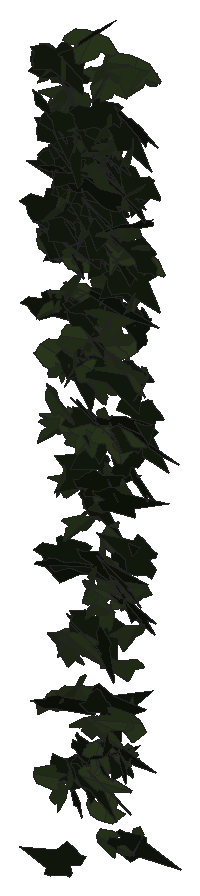
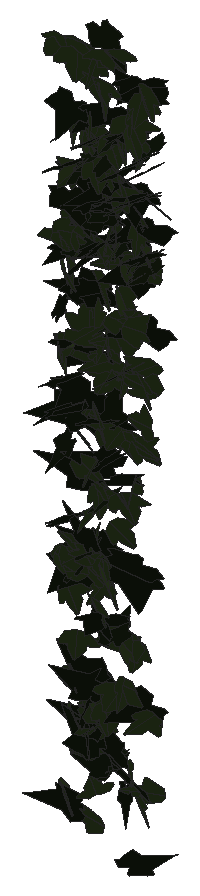
# SketchUp Ruby script. Lengths in millimetres.
U = 1.mm
M = Sketchup.active_model
def pt(a) = Geom::Point3d.new(a.map { |v| v * U })
def face(e, loops, mat)
  f = e.add_face(loops[0].map { |a| pt(a) })
  loops[1..].each { |l| e.add_face(l.map { |a| pt(a) }).erase! }
  f.material = f.back_material = mat if mat
  f
end
# faces: each face lists its corners as indices into pts; further lists are holes
def faces(e, pts, list, mat = nil) = list.each { |f| face(e, (f[0].is_a?(Array) ? f : [f]).map { |l| l.map { |i| pts[i] } }, mat) }
# xy, xz, yz: faces in a plane at the given z, y or x. An outline is a flat list of corners, or four numbers for a rectangle; further outlines are holes
def ring(l) = l.size == 4 ? [[l[0], l[1]], [l[2], l[1]], [l[2], l[3]], [l[0], l[3]]] : l.each_slice(2).to_a
def flat(e, list, mat, &to3) = list.each { |f| face(e, (f[0].is_a?(Array) ? f : [f]).map { |l| ring(l).map { |u, v| to3.(u, v) } }, mat) }
def xy(e, z, list, mat = nil) = flat(e, list, mat) { |x, y| [x, y, z] }
def xz(e, y, list, mat = nil) = flat(e, list, mat) { |x, z| [x, y, z] }
def yz(e, x, list, mat = nil) = flat(e, list, mat) { |y, z| [x, y, z] }
def lines(e, pts, list) = list.each { |a, b| e.add_line(pt(pts[a]), pt(pts[b])) }
# prism: a flat outline (further loops are holes) pulled along v
def prism(e, loops, v, mat = nil)
  f = face(e, loops, mat); d = Geom::Vector3d.new(v.map { |x| x * U })
  f.pushpull(f.normal.samedirection?(d) ? d.length : -d.length)
end
def box(e, o, s, mat = nil) = prism(e, [[o, [o[0] + s[0], o[1], o[2]], [o[0] + s[0], o[1] + s[1], o[2]], [o[0], o[1] + s[1], o[2]]]], [0, 0, s[2]], mat)
def at(x, y, z, deg = 0) = Geom::Transformation.translation(pt([x, y, z])) * Geom::Transformation.rotation(ORIGIN, Z_AXIS, deg.degrees)
def axes(o, x, y, z) = Geom::Transformation.new([*x, 0, *y, 0, *z, 0, *pt(o).to_a, 1])
def part(name) = M.definitions.add(name)
# library, detail: a bought-in or finely detailed component or shape, given as its bounding box
def library(name, o, s) = part(name).tap { |d| box(d.entities, o, s) }
def detail(e, o, s) = box(e.add_group.entities, o, s)
def put(e, d, t, mat = nil) = e.add_instance(d, t).tap { |i| i.material = mat if mat }
def group(e, t, mat = nil) = e.add_group.tap { |g| g.transformation = t; g.material = mat if mat }.entities
root = M.entities
M.materials.add("efeu1").color = [18, 25, 13]
M.materials.add("efeu2").color = [43, 57, 29]
c1 = part("ivyleaf_9")
p = [[39.1,54.8,31.7],[34.5,51.8,30.2],[-5.3,25.2,17.3],[-17.9,28.3,20.9],[-21.6,21.7,17],[-20.2,4.3,5.3],
  [-22.9,-0.3,2.5],[-17.1,-4,-0.6],[-2,-2.1,-1.2],[-0.7,-15.4,-10.1],[16.6,-22.3,-16.7],[21.1,-15.1,-12.5],
  [32.7,-10.7,-11],[46.1,-1.8,-6.6],[30.8,11.2,3.8]]
faces(c1.entities,p,[[0,1,2,3,4,5,6,7,8,9,10,11,12,13,14]],"efeu1")
c2 = part("ivyleaf_10")
p = [[0,12.8,-0.8],[-1.5,51.3,-10.9],[-4.9,51,-11.6],[-13.6,26.5,-7.3],[-13.2,15.9,-4.6],[-21.1,19.3,-7.2],
  [-29.5,16.3,-8.3],[-29.2,8.3,-6.2],[-19.7,-9.8,0.5],[-7.6,-13,4],[1,-12.2,5.8],[-0.4,51.1,-11.1],
  [-1.5,51.1,-10.9],[1,-12.4,5.9],[16.9,-12.4,3.5],[35.1,9.1,-5.1],[35,12.9,-6.1],[20.5,16.4,-4.9],
  [15.8,15,-3.8],[15.3,27.6,-7.1],[12.8,31.3,-7.8]]
faces(c2.entities,p,[[0,1,2,3,4,5,6,7,8,9,10],[11,12,0,13,14,15,16,17,18,19,20]],"efeu2")
put(root,c1,axes([2017.3,949.6,846.8],[0.22313,0.05004,0.79873],[1.37801,0.33725,-0.12741],[-0.64884,0.73347,0.00409]))
put(root,c2,axes([2051.2,960.3,1148.2],[-1.33642,-0.23546,0.06145],[-0.10791,-0.0242,-0.74061],[0.45038,-0.70447,0.00491]))
put(root,c2,axes([2099.1,965.4,1580.9],[-1.10747,-0.55056,0.2142],[-0.17202,-0.21415,-0.79598],[1.11111,-0.58192,0.09026]))
put(root,c2,axes([2088.2,957.8,1448.8],[0.19663,-0.77036,-0.31589],[0.05218,0.32128,-0.77456],[1.58377,0.08505,0.06474]))
put(root,c2,axes([1923,963.4,1232.1],[-0.03515,-0.04676,0.81979],[1.56112,0.03653,0.02056],[-0.07163,0.81918,0.04588]))
put(root,c1,axes([1995,969.1,336.1],[0.64527,-0.78076,0.06942],[0.0749,-0.05858,-0.85111],[1.48993,0.34108,0.01272]))
put(root,c2,axes([1955,966.6,1335.6],[0.91903,-0.61856,0.09808],[0.10345,-0.08199,-0.78469],[1.18745,0.48588,-0.00755]))
put(root,c2,axes([2072.5,963.3,1299.6],[-0.8108,-0.67903,0.04435],[-0.04819,-0.03647,-0.8016],[1.29418,-0.42676,-0.00206]))
put(root,c2,axes([2086.8,962.5,459.6],[0.64898,-0.00928,-0.69136],[-1.3048,0.09545,-0.33942],[0.17068,0.76495,0.03397]))
put(root,c1,axes([2016.9,971.5,582.5],[-0.39013,0.04915,-0.84771],[1.57044,-0.19423,-0.2108],[-0.38131,-0.85024,-0.00085]))
put(root,c2,axes([2013.5,964.2,432],[-0.80071,0.13176,-0.54735],[0.98165,-0.18367,-0.44067],[-0.42945,-0.66548,0.01325]))
put(root,c1,axes([2055.7,980,1208.8],[0.36229,-0.31801,-0.71542],[0.61667,-0.63825,0.36992],[-1.35645,-0.3751,-0.02291]))
put(root,c2,axes([2037.4,962.1,1436.9],[-0.52323,-0.77628,-0.1375],[0.09712,0.12779,-0.82351],[1.49727,-0.27956,0.00536]))
put(root,c1,axes([2008.8,973.2,945.6],[1.07179,-0.67128,0.12791],[-0.10135,0.12214,0.87542],[-1.29661,-0.56443,0.03731]))
put(root,c2,axes([1942.4,973.1,919.2],[-0.2544,-0.58614,0.47424],[-0.23255,-0.45842,-0.60103],[1.41597,-0.1806,-0.01351]))
put(root,c1,axes([1949.1,957.5,1529.6],[-0.86966,-0.09896,0.70036],[1.33591,0.03932,0.46352],[-0.16592,0.83532,0.06115]))
put(root,c1,axes([2004.6,963.6,1339.3],[0.22572,-0.16988,0.8106],[1.48383,-0.25337,-0.16717],[0.53179,0.77907,0.12239]))
put(root,c1,axes([1980.2,966.9,1133.4],[0.57441,-0.71253,-0.15559],[-0.05756,0.15602,-0.77314],[1.38685,0.30159,0.03235]))
put(root,c2,axes([1938.2,953.1,1054.1],[0.51783,0.45753,0.6261],[0.58708,0.5449,-0.53225],[-1.35405,0.41123,0.00867]))
put(root,c1,axes([1956.2,973.8,164.7],[-0.09001,-0.01374,0.76617],[-1.35631,-0.28136,-0.04904],[0.53606,-0.7142,0.00458]))
put(root,c2,axes([2007.8,958.4,340.2],[-0.27323,-0.14885,-0.75209],[1.39735,0.19361,-0.17847],[0.42011,-0.74078,0.10448]))
put(root,c1,axes([1983.4,974.7,1025.8],[-0.02468,-0.76983,0.10528],[-0.00828,-0.10522,-0.76993],[1.47875,-0.01344,-0.00255]))
put(root,c1,axes([1943.6,963.3,1565.4],[-0.2483,-0.62877,-0.56176],[0.14015,0.55778,-0.64141],[1.59858,-0.14656,-0.03102]))
put(root,c1,axes([2040.6,971.7,474.3],[-0.10227,-0.21449,0.73979],[1.00549,-0.54991,-0.12106],[1.06677,0.49777,0.18503]))
put(root,c1,axes([2002.5,975.7,1317.4],[0.41487,-0.64149,0.45015],[0.41534,-0.39907,-0.67437],[1.43249,0.30149,0.06516]))
put(root,c2,axes([1959.7,959.8,550.7],[-1.33318,0.37854,0.14958],[-0.25108,0.07051,-0.79623],[-0.73283,-0.71281,0.00068]))
put(root,c2,axes([1924.4,973.5,961.1],[0.23048,-0.23441,0.79724],[1.40468,-0.33987,-0.21204],[0.72674,0.73127,0.15701]))
put(root,c1,axes([1974,965.2,1275.6],[-0.38098,-0.57923,-0.54341],[0.42026,0.49772,-0.61187],[1.45199,-0.29604,0.03452]))
put(root,c1,axes([1915.1,977.1,1456.4],[0.2872,-0.68165,0.39536],[0.20986,-0.38032,-0.6978],[1.48498,0.18558,0.02215]))
put(root,c1,axes([1928.9,957.3,1309.3],[-0.00385,-0.34703,-0.79748],[0.39652,0.77407,-0.33738],[1.60704,-0.19182,0.08133]))
put(root,c2,axes([2004.8,974,926.9],[-0.48843,-0.595,0.42459],[-0.03561,-0.4445,-0.63422],[1.39071,-0.22035,0.13288]))
put(root,c2,axes([1978.2,952,1093.1],[-0.2951,-0.17635,-0.85934],[1.20506,0.5815,-0.23358],[1.15556,-0.65144,0.02413]))
put(root,c1,axes([2038.5,972.1,708],[0.68577,-0.65111,0.19844],[0.18153,-0.17402,-0.74416],[1.28269,0.37273,-0.00078]))
put(root,c1,axes([2059.5,977.7,1364.5],[0.17038,-0.6586,0.46324],[0.40942,-0.42959,-0.65233],[1.47676,0.19509,0.12741]))
put(root,c2,axes([1999.8,962.3,922.1],[0.98723,-0.29665,-0.41728],[-0.63076,0.25821,-0.59555],[0.7427,0.61362,0.04888]))
put(root,c1,axes([1974.7,958.9,1371.3],[-0.88416,0.53391,0.36751],[-0.53638,0.24078,-0.70607],[-1.11087,-0.54121,0.04842]))
put(root,c2,axes([1984.1,977.6,1327.7],[0.17658,-0.30387,0.75573],[1.04993,-0.53617,-0.28332],[1.14055,0.54062,0.1438]))
put(root,c2,axes([2052.2,965.3,943.1],[1.37774,0.28758,0.14692],[0.26326,0.04974,-0.77892],[-0.55538,0.73699,-0.00476]))
put(root,c1,axes([1939,952.2,451],[1.26595,0.38495,0.3228],[0.50845,0.18255,-0.76821],[-0.80974,0.71647,0.02229]))
put(root,c2,axes([2027.8,974,943],[0.36732,-0.19282,0.66763],[1.10294,-0.33772,-0.26507],[0.72987,0.60739,0.06456]))
put(root,c1,axes([2054.6,981.6,1238.4],[-0.1307,-0.54907,0.63036],[0.24748,-0.63181,-0.53616],[1.57164,0.05383,0.13685]))
put(root,c2,axes([1960.7,957.1,841.4],[0.15558,-0.60823,-0.51662],[0.22322,0.52284,-0.597],[1.50231,-0.0147,0.14221]))
put(root,c1,axes([2066.6,982,654.5],[-0.02983,-0.43981,0.68525],[0.02123,-0.68543,-0.43967],[1.54952,0.00093,0.01922]))
put(root,c1,axes([2023.6,963.3,1630.6],[-0.396,0.75605,-0.28918],[0.176,-0.27443,-0.78401],[-1.53049,-0.22718,-0.01533]))
put(root,c2,axes([2057.4,979.8,1260.9],[-0.16097,-0.55649,0.62678],[0.35005,-0.62693,-0.53181],[1.55633,0.08345,0.18444]))
put(root,c2,axes([2033.6,963,1378.6],[-1.4652,0.10412,0.33772],[-0.64465,0.01357,-0.77632],[-0.1919,-0.84057,0.0293]))
put(root,c1,axes([2053.6,975.7,1166.6],[-0.0147,-0.02878,-0.80378],[-0.64011,-0.73005,0.02937],[-1.39048,0.33638,-0.00502]))
put(root,c2,axes([2046.2,971.1,1434.8],[-0.00868,-0.80127,0.13001],[-0.03442,-0.12988,-0.8011],[1.54454,-0.0074,-0.01712]))
put(root,c2,axes([2083.9,969.9,615.8],[-0.41394,-0.75893,0.10008],[-0.0215,-0.10085,-0.7893],[1.45674,-0.21714,0.01679]))
put(root,c1,axes([2009.8,967.5,1446.6],[0.63071,-0.69883,-0.2613],[0.06158,0.29911,-0.75891],[1.41861,0.29771,0.14911]))
put(root,c2,axes([2044.7,972.4,1097.9],[-0.94798,-0.6166,-0.17507],[-0.20852,-0.13655,0.79266],[-1.20195,0.51001,0.00057]))
put(root,c2,axes([1977.5,974.3,1445.4],[0.46495,-0.70608,0.29635],[0.34947,-0.24797,-0.74219],[1.41486,0.29328,0.08593]))
put(root,c1,axes([1933.9,965.7,1240.9],[0.65194,-0.65099,-0.38619],[-0.27509,0.35984,-0.73478],[1.41407,0.37013,0.03511]))
put(root,c2,axes([1950.2,965.2,1035],[0.89916,-0.6454,-0.29145],[-0.28808,0.25022,-0.79948],[1.31661,0.49552,0.02411]))
put(root,c2,axes([1947.7,982,1130.8],[-0.13574,-0.4363,0.75754],[-0.22223,-0.74849,-0.44209],[1.64887,-0.1368,0.00278]))
put(root,c1,axes([2011.4,971.9,700.2],[0.48049,-0.22291,0.73659],[1.12002,-0.44362,-0.33595],[0.94382,0.63992,0.02368]))
put(root,c2,axes([1966.7,967.8,563.1],[-0.98505,0.14037,-0.65553],[1.19464,-0.18934,-0.53614],[-0.44803,-0.81348,0.01168]))
put(root,c1,axes([2025.3,974.1,1315],[-1.25694,-0.28531,-0.38832],[0.70404,0.12198,-0.71878],[0.58769,-0.75637,0.03056]))
put(root,c1,axes([2025.5,965.6,1163],[1.06675,-0.13073,0.50882],[0.92625,-0.15095,-0.5749],[0.37649,0.74181,-0.02732]))
put(root,c1,axes([1954.1,980.3,1238.6],[0.22312,-0.67059,0.38038],[0.08005,-0.37861,-0.68045],[1.46511,0.12281,-0.02075]))
put(root,c2,axes([1930.5,970.9,1266.9],[0.57811,-0.70834,0.0458],[0.04705,-0.03923,-0.77069],[1.35011,0.30468,0.00725]))
put(root,c1,axes([1968,960.2,1366.3],[0.96449,0.45524,-0.40751],[-0.73472,-0.17179,-0.672],[-0.90131,0.62719,0.11172]))
put(root,c1,axes([1983.6,975.7,1338.3],[-0.51996,-0.74959,-0.16478],[0.08137,0.15977,-0.79769],[1.45841,-0.27616,-0.01424]))
put(root,c2,axes([2010.3,965.5,1020.2],[-1.34199,0.14114,-0.10133],[0.1947,-0.00507,-0.71895],[-0.26728,-0.71235,-0.01496]))
put(root,c2,axes([2008.2,962.4,1043.4],[-0.62937,-0.33628,-0.58463],[1.0408,0.24739,-0.45163],[0.75127,-0.62446,0.13591]))
put(root,c1,axes([2074.6,965.2,1227.1],[0.05079,-0.53096,-0.58579],[0.14023,0.58524,-0.5271],[1.49813,-0.03678,0.0692]))
put(root,c1,axes([1966.2,965,1462.8],[0.24546,-0.58757,-0.57627],[0.02116,0.5845,-0.59347],[1.56619,0.08419,0.09833]))
put(root,c2,axes([2068.5,972,1046.7],[-1.36516,-0.11572,-0.25862],[-0.48066,-0.05795,0.7264],[-0.24443,0.76029,0.016]))
put(root,c1,axes([1923.3,959.6,1131.9],[-0.01897,-0.00816,-0.79816],[0.68922,0.7113,-0.01179],[1.3538,-0.36224,-0.00518]))
put(root,c1,axes([1986.4,984.1,329.6],[0.0063,-0.62618,0.51013],[-0.0175,-0.51013,-0.62612],[1.53707,-0.00324,-0.00922]))
put(root,c2,axes([2085.2,970.9,1590.1],[1.60703,-0.03795,0.0025],[0.00622,0.01701,-0.84506],[0.07211,0.84422,0.01714]))
put(root,c1,axes([2024.7,974.6,1326.6],[-0.13993,-0.74961,-0.20474],[-0.01798,0.2065,-0.75267],[1.47881,-0.06842,-0.02853]))
put(root,c1,axes([1985.6,978.8,1127.3],[0.23018,-0.86457,0.05842],[0.01918,-0.05758,-0.87298],[1.64909,0.12135,0.002]))
put(root,c2,axes([1962.6,960.9,1517.1],[-0.52422,0.69997,0.30219],[-0.28112,0.26623,-0.7513],[-1.42354,-0.31034,0.03709]))
put(root,c2,axes([1997.2,962.5,1279.7],[0.3284,-0.71204,-0.44932],[0.01499,0.46,-0.72594],[1.60233,0.14163,0.09888]))
put(root,c2,axes([2046.2,972,1443.6],[1.01335,-0.61331,-0.0153],[-0.02349,0.00955,-0.81218],[1.16737,0.53258,-0.00306]))
put(root,c1,axes([1935.1,981,1263.3],[-0.30244,-0.73599,0.14313],[0.03223,-0.14979,-0.75147],[1.42662,-0.15265,0.04732]))
put(root,c2,axes([1949.5,964,1297.6],[-0.31592,-0.69127,-0.35294],[0.14364,0.34484,-0.71089],[1.47018,-0.18223,-0.00639]))
put(root,c1,axes([2084.6,964.6,1316.3],[0.07682,0.75873,-0.26869],[-0.09153,-0.26628,-0.75913],[-1.52915,0.05405,0.03194]))
put(root,c2,axes([1939.3,965.9,1552.8],[1.09786,-0.50635,-0.3483],[-0.26976,0.3552,-0.75113],[1.13812,0.57262,0.15794]))
put(root,c2,axes([2074.3,973.4,397.6],[0.67773,-0.68384,0.05504],[0.06154,-0.04521,-0.77096],[1.30424,0.35748,0.00777]))
put(root,c2,axes([2007.4,965.4,1096.5],[0.17011,-0.76116,-0.33495],[0.08463,0.34077,-0.76252],[1.58043,0.06368,0.07688]))
put(root,c1,axes([2040.9,962,828.7],[0.99141,0.35781,-0.5095],[0.50999,0.47078,0.60459],[1.06954,-0.55616,0.18399]))
put(root,c2,axes([2039.2,962.6,1472],[-0.0133,-0.65575,-0.47411],[0.13895,0.47168,-0.65347],[1.53376,-0.04842,0.05509]))
put(root,c1,axes([2054.9,958.8,972.3],[1.25908,0.41069,0.14511],[0.2166,0.09173,-0.77847],[-0.80018,0.67105,0.01761]))
put(root,c1,axes([2003.1,978.8,330.8],[0.71686,-0.56346,0.39178],[0.43516,-0.31835,-0.67766],[1.23151,0.44048,0.0114]))
put(root,c2,axes([1982.3,979.4,763],[-0.30692,-0.62162,0.40611],[-0.17057,-0.39624,-0.6421],[1.40283,-0.18418,0.01078]))
put(root,c2,axes([2084.7,967.2,1192.3],[0.33257,-0.73806,-0.29627],[0.0382,0.30734,-0.75378],[1.51314,0.15446,0.08414]))
put(root,c1,axes([2051.6,973.7,1056.5],[-0.80539,-0.46487,-0.6064],[0.8238,0.42538,-0.62817],[1.19836,-0.60485,0.02428]))
put(root,c2,axes([1961.8,980.1,559.3],[0.0504,-0.64237,0.38785],[0.03877,-0.38733,-0.6429],[1.42759,0.0332,0.00377]))
put(root,c1,axes([1985.9,984.5,850.6],[-0.88152,-0.51274,0.32806],[-0.42432,-0.24069,-0.69096],[1.078,-0.51403,-0.00371]))
put(root,c1,axes([2003.9,984.2,1300.6],[0.06445,-0.50671,0.63045],[0.57057,-0.5782,-0.48081],[1.42974,0.25358,0.16346]))
put(root,c1,axes([1970,973.4,1269.1],[0.84925,-0.62635,-0.09543],[-0.08243,0.08629,-0.7689],[1.203,0.44808,0.01468]))
put(root,c1,axes([2012.5,963.1,1491.2],[-0.05861,-0.3485,-0.76476],[0.06546,0.76411,-0.34959],[1.59816,-0.04408,-0.01373]))
put(root,c2,axes([2036.1,965.7,1078.9],[-1.14068,0.31923,0.27874],[-0.45876,0.14031,-0.67899],[-0.66339,-0.64593,-0.00973]))
put(root,c2,axes([1956.9,966.2,1502.8],[-0.15118,-0.74912,-0.37046],[0.18575,0.36127,-0.75146],[1.57965,-0.11417,0.05291]))
put(root,c1,axes([1973.9,984.4,1400.9],[-0.33434,-0.77637,0.16821],[-0.11239,-0.15904,-0.7957],[1.5077,-0.18402,-0.02201]))
put(root,c2,axes([2020.5,962.7,640.3],[-0.30163,-0.47046,-0.53826],[0.45016,0.48577,-0.49423],[1.28394,-0.28084,0.04683]))
put(root,c2,axes([1976.8,959.4,1035],[0.06562,-0.53503,-0.71444],[0.06378,0.71524,-0.53402],[1.69754,-0.00619,0.04768]))
put(root,c1,axes([2044.4,987.5,377.6],[-0.24088,-0.54335,0.52327],[-0.10946,-0.52209,-0.55604],[1.4315,-0.13135,0.04553]))
put(root,c1,axes([2067.6,966,660.8],[1.54528,-0.0685,-0.22433],[-0.42506,0.02115,-0.81482],[0.13638,0.84209,0.00222]))
put(root,c2,axes([1970.8,960.2,328.5],[0.07035,-0.13669,-0.67879],[-0.3157,0.65822,-0.14158],[1.27943,0.16993,0.00239]))
put(root,c2,axes([1983.9,980.7,1078],[-0.04186,0.0285,0.83238],[1.44658,-0.33976,0.03172],[0.64809,0.7602,-0.01703]))
put(root,c1,axes([1984.7,983.8,565.5],[0.87522,-0.63846,-0.0692],[0.08935,-0.05147,0.78679],[-1.21896,-0.46219,0.00798]))
put(root,c2,axes([2000.2,962.3,1285],[0.05694,-0.61439,-0.60164],[0.24945,0.59823,-0.60439],[1.61746,-0.07063,0.11439]))
put(root,c2,axes([2067.2,971.2,449.7],[0.78539,-0.64616,0.10611],[-0.10984,0.08905,0.7667],[-1.2414,-0.41668,-0.00071]))
put(root,c2,axes([1979,958.1,1225.5],[-0.04263,-0.11945,0.83068],[0.44668,0.79693,0.12092],[-1.53349,0.23545,0.01213]))
put(root,c2,axes([1995,975.6,1444.5],[-0.58946,-0.76156,0.08257],[0.02244,-0.09379,-0.82084],[1.45772,-0.30651,0.04602]))
put(root,c2,axes([2021.3,969.1,378],[0.66793,-0.02681,-0.67078],[1.2734,0.07563,0.34704],[0.10408,-0.75325,0.05872]))
put(root,c1,axes([1956.9,966.6,686.5],[0.82423,0.58831,-0.33978],[-0.40268,-0.26612,-0.73043],[-1.2287,0.48186,0.01145]))
put(root,c2,axes([2088.5,983.3,676],[-0.05393,-0.49828,0.49008],[-0.07797,-0.48845,-0.499],[1.32786,-0.04892,-0.0094]))
put(root,c2,axes([1971.5,977.2,1178.7],[0.08405,-0.92118,0.08716],[0.02857,-0.08654,-0.92217],[1.76078,0.04537,0.0108]))
put(root,c1,axes([2030.2,977,396.8],[0.76971,0.01153,-0.68215],[1.28542,0.1053,0.4022],[0.18349,-0.786,0.04388]))
put(root,c2,axes([1958.6,976.5,1491.9],[-1.1208,-0.54754,0.16804],[-0.09561,-0.19071,-0.79746],[1.08584,-0.58196,0.10323]))
put(root,c1,axes([1966.7,971.7,1045.4],[0.55834,-0.65262,-0.41026],[-0.10485,0.42009,-0.70766],[1.46335,0.2791,0.10583]))
put(root,c2,axes([1940.3,966.9,1533.7],[-0.4526,-0.69392,-0.40727],[0.25869,0.38394,-0.73353],[1.50933,-0.27389,0.0036]))
put(root,c2,axes([2037.1,978.6,696.7],[-0.44603,-0.09509,0.77883],[1.47644,-0.1498,0.21515],[0.22361,0.79941,0.13295]))
put(root,c2,axes([1997.9,975.9,1601.4],[1.31023,0.41131,-0.22014],[-0.3839,-0.0914,-0.80159],[-0.80059,0.71697,0.0241]))
put(root,c2,axes([2026.7,977.7,384.2],[0.96279,0.59729,-0.32327],[-0.423,-0.2353,-0.78257],[-1.22141,0.55232,0.0162]))
put(root,c2,axes([2065.5,972.1,1575.5],[-1.24533,-0.52079,-0.06307],[0.08631,0.04429,-0.83626],[0.99466,-0.65587,-0.0064]))
put(root,c2,axes([2091.9,974,258.9],[0.53858,-0.73749,-0.12828],[-0.07825,0.12162,-0.7899],[1.42252,0.28591,0.00512]))
put(root,c2,axes([2031.4,964.7,1568.9],[-0.08983,-0.62052,-0.55209],[0.28539,0.53752,-0.61697],[1.55476,-0.13452,0.08135]))
put(root,c1,axes([2085.7,959.9,904.1],[-0.26286,0.5301,0.62137],[-0.39012,0.58752,-0.54679],[-1.50472,-0.24493,0.03322]))
put(root,c1,axes([2103.1,984.4,1257.8],[-0.06801,-0.7717,-0.11443],[0.03996,-0.11546,0.77209],[-1.48422,0.03225,0.02603]))
put(root,c2,axes([2007.1,970.6,653.7],[0.65541,-0.55506,-0.34467],[-0.28951,0.31079,-0.6525],[1.20932,0.37523,0.03059]))
put(root,c2,axes([2090.8,986.7,1257.1],[0.05684,0.15929,-0.76146],[-0.83547,-0.62565,-0.1481],[-1.22232,0.43505,0.06582]))
put(root,c2,axes([1947.2,969.2,289.9],[0.57275,-0.59491,-0.43946],[-0.36781,0.39472,-0.66668],[1.35875,0.35762,0.00478]))
put(root,c1,axes([1923.2,981,1420.1],[0.19809,-0.80532,-0.11078],[0.00388,0.11194,-0.81186],[1.54712,0.10283,0.01622]))
put(root,c1,axes([2005.7,981.9,943.7],[-0.74361,-0.68212,-0.24032],[0.24058,0.20453,-0.78606],[1.35523,-0.41059,0.00768]))
put(root,c1,axes([1941.2,988.1,1364.2],[-0.4262,-0.72771,0.22445],[-0.06433,-0.22422,-0.76071],[1.44794,-0.22416,0.03227]))
put(root,c2,axes([1922.2,970.8,1025.5],[-0.45797,-0.31336,0.59718],[0.98478,0.32086,0.37686],[-0.82317,0.55819,0.11862]))
put(root,c2,axes([2063.6,981.6,659.6],[-0.27222,-0.0674,-0.69603],[-1.22931,-0.25949,0.15786],[-0.50995,0.6615,-0.00899]))
put(root,c1,axes([1936.1,986,1434.7],[-0.1041,-0.79723,0.10403],[-0.04271,-0.10271,-0.79896],[1.52955,-0.05712,-0.01523]))
put(root,c2,axes([2024.1,976.5,1541.9],[1.52464,-0.17079,-0.0484],[-0.07163,0.05522,-0.8178],[0.33018,0.80065,0.04608]))
put(root,c1,axes([1942.6,971.2,707.7],[0.14518,-0.23519,-0.81969],[1.06466,0.63495,-0.13012],[1.22498,-0.52398,0.21024]))
put(root,c1,axes([2097.7,985.3,736],[-0.38876,-0.77888,-0.18429],[-0.08959,-0.17818,0.80522],[-1.52066,0.20962,-0.00033]))
put(root,c1,axes([2035.1,989.2,423.3],[0.01208,-0.07896,-0.77377],[0.95,-0.59301,0.06461],[-1.13523,-0.49709,0.04583]))
put(root,c2,axes([2022.9,973.1,810.8],[-0.34976,-0.73893,-0.18809],[0.04618,0.18771,-0.76114],[1.45043,-0.18416,-0.02112]))
put(root,c2,axes([1915.4,966.4,306.8],[0.05848,-0.04265,0.68193],[0.81393,0.53357,0.0141],[-1.01417,0.42576,0.05063]))
put(root,c2,axes([1968.2,984.4,1360.4],[-0.34941,-0.65614,0.39725],[-0.07899,-0.39937,-0.67883],[1.45766,-0.17892,0.05844]))
put(root,c1,axes([1926.3,978.7,1237.9],[0.51778,-0.69458,-0.17136],[-0.0547,0.17257,-0.74513],[1.36046,0.27129,0.03526]))
put(root,c1,axes([1988.1,985.4,1451.3],[0.4551,-0.76209,0.16662],[0.05561,-0.1654,-0.79845],[1.48363,0.23997,-0.02118]))
put(root,c2,axes([2029.5,979.9,412.8],[0.09117,-0.78449,-0.11342],[0.06241,-0.11157,0.78553],[-1.50728,-0.05207,0.02567]))
put(root,c2,axes([2016.8,972.4,1527.9],[0.28295,-0.77014,-0.30489],[-0.03404,0.30671,-0.78345],[1.57605,0.14489,0.03782]))
put(root,c1,axes([2014.4,986.8,1419.8],[0.1962,-0.77423,0.18754],[0.11504,-0.18095,-0.78028],[1.51176,0.11425,0.03504]))
put(root,c2,axes([2001.7,985.2,684.4],[0.37282,-0.70049,0.35531],[0.23704,-0.33386,-0.72687],[1.47596,0.23056,0.02699]))
put(root,c1,axes([2026.6,991.4,1235.9],[-0.89836,-0.54266,0.27252],[-0.05035,-0.32646,-0.6959],[1.15462,-0.43646,0.18169]))
put(root,c1,axes([1998.5,979.9,1411.8],[0.95628,-0.62396,-0.03767],[-0.05994,0.02299,-0.80105],[1.18816,0.50334,-0.0101]))
put(root,c1,axes([2006.8,963.2,1346.7],[0.3619,-0.00504,-0.81571],[-0.03747,0.83731,-0.00976],[1.55204,0.02139,0.18997]))
put(root,c2,axes([2003.8,976.5,429.4],[-0.68754,-0.66782,-0.07811],[0.06839,0.06937,-0.75926],[1.27783,-0.36303,-0.00139]))
put(root,c2,axes([2012.9,987.7,735.7],[0.36359,-0.44079,0.55727],[0.71307,-0.42782,-0.46684],[1.14898,0.40499,0.11338]))
put(root,c2,axes([1964,982.7,1145.5],[0.54052,0.5147,-0.46604],[-0.73741,-0.30035,-0.56783],[-1.09659,0.45568,0.15212]))
put(root,c2,axes([1956.3,987.4,1244.8],[0.09757,-0.63069,0.43616],[0.22589,-0.42534,-0.62899],[1.44182,0.10932,0.06903]))
put(root,c1,axes([1927.3,986,1267.4],[-0.27744,-0.75355,-0.06555],[0.01273,0.06547,-0.7675],[1.43952,-0.14581,-0.00585]))
put(root,c1,axes([2078.8,991.3,1381.9],[-0.46948,-0.75446,0.21526],[-0.07613,-0.21326,-0.7933],[1.49125,-0.24841,0.02727]))
put(root,c2,axes([1974.4,968.5,479.7],[-0.26735,-0.63503,-0.53464],[0.15062,0.52952,-0.64975],[1.57269,-0.15866,-0.02866]))
put(root,c2,axes([1969,975.2,922.2],[-0.1324,0.16608,0.73125],[-1.42711,-0.02178,-0.06639],[0.01239,-0.73423,0.16738]))
put(root,c1,axes([2061.1,968.1,388.2],[0.35739,-0.03822,-0.76001],[-1.36058,0.25941,-0.18968],[0.49632,0.73864,0.02729]))
put(root,c1,axes([1970.6,985.2,371.6],[0.28146,-0.08299,-0.76379],[1.45627,-0.05412,0.15403],[-0.13165,-0.77609,0.07094]))
put(root,c1,axes([1911,988.7,1243.8],[0.35819,-0.71251,0.29751],[0.25875,-0.27085,-0.73468],[1.44655,0.22488,0.05775]))
put(root,c1,axes([2015.9,978.4,1258.7],[0.2906,-0.67184,-0.37989],[-0.07388,0.38008,-0.68777],[1.46704,0.15222,0.04061]))
put(root,c2,axes([2020.2,983.4,227],[0.01079,0.00174,-0.68587],[1.10022,-0.36912,0.00385],[-0.70246,-0.5781,-0.00452]))
put(root,c2,axes([2101.4,973.8,1049.9],[0.34628,-0.75957,-0.40544],[-0.21759,0.38941,-0.78085],[1.62416,0.21412,-0.01817]))
put(root,c1,axes([1993,980.6,1271.2],[0.29563,-0.693,-0.30453],[-0.09157,0.30121,-0.70998],[1.43774,0.16168,0.0174]))
put(root,c1,axes([2062.1,975.8,243.3],[0.37516,0.03102,-0.74405],[1.13332,0.45561,0.17676],[0.85107,-0.62039,0.0926]))
put(root,c2,axes([2039.8,967.4,763.7],[-0.14916,0.44545,0.52663],[-0.15195,0.5206,-0.45223],[-1.30392,-0.11162,-0.00754]))
put(root,c2,axes([1976.8,977.4,934.9],[1.31231,0.36327,0.25308],[0.40472,0.13908,-0.77903],[-0.73904,0.72122,0.02276]))
put(root,c1,axes([2056.8,978.8,1463.7],[0.60613,-0.67457,-0.37044],[-0.28779,0.33825,-0.74594],[1.43615,0.35249,0.00687]))
put(root,c1,axes([2085.1,988.1,997.2],[-0.18807,-0.75434,-0.03692],[0.00915,0.0366,-0.76079],[1.43735,-0.09893,0.00001]))
put(root,c2,axes([2011.7,984.9,667.4],[-0.68929,0.10231,0.74224],[1.36421,-0.19271,0.37632],[0.41516,0.80309,-0.00425]))
put(root,c2,axes([1979.8,976.2,471.6],[-1.22781,-0.34514,-0.25102],[0.42745,0.11231,-0.73162],[0.69066,-0.68307,0.00655]))
put(root,c1,axes([1995.9,980.7,810.5],[0.76619,-0.70404,-0.26185],[-0.2228,0.23465,-0.81089],[1.41214,0.41902,0.01414]))
put(root,c2,axes([1984.9,979.2,1262],[-0.34469,0.74708,-0.10848],[0.05311,-0.10486,-0.76872],[-1.43577,-0.18323,-0.00239]))
put(root,c2,axes([2077,983.7,672.6],[-1.04135,-0.09519,-0.47966],[-0.90299,-0.07095,0.55531],[-0.22535,0.72417,-0.00864]))
put(root,c1,axes([2018.7,989.4,1447.8],[-0.01812,-0.80788,0.00172],[0.00062,-0.00172,-0.80794],[1.53756,-0.00952,0.00034]))
put(root,c2,axes([2021.1,978.7,952.2],[0.57466,-0.67464,-0.22854],[-0.10478,0.22538,-0.73805],[1.35159,0.30431,0.03996]))
put(root,c2,axes([2080.6,964.8,1359.2],[0.40227,0.13712,0.75103],[-0.34591,0.76591,-0.08868],[-1.41121,-0.14865,0.23582]))
put(root,c2,axes([1923.2,970.2,438.7],[-0.49896,-0.36271,-0.63131],[0.70621,0.51075,-0.44754],[1.19224,-0.45433,0.00089]))
put(root,c1,axes([1969.3,972.4,296.7],[0.57675,-0.1444,-0.69135],[-1.20971,0.27223,-0.33547],[0.58603,0.70406,-0.01209]))
put(root,c2,axes([1967.5,985.5,1383.1],[0.74241,-0.68075,0.16164],[0.30181,-0.09423,-0.77954],[1.29698,0.4116,0.08887]))
put(root,c2,axes([1924.6,979,1452.2],[-0.54627,0.74356,-0.07563],[0.06655,-0.06757,-0.79699],[-1.42088,-0.28903,-0.00825]))
put(root,c2,axes([2024.3,981.5,1394.8],[-0.50163,-0.77427,-0.03397],[0.00973,0.03415,-0.81788],[1.47498,-0.26355,-0.00616]))
put(root,c1,axes([2081,974.7,881],[1.06388,-0.33466,-0.50134],[-0.77418,0.29514,-0.65057],[0.8466,0.69044,0.0351]))
put(root,c2,axes([2018.6,981.7,697.2],[-0.74538,0.08832,-0.63245],[1.16213,-0.16536,-0.40122],[-0.35573,-0.72528,0.01446]))
put(root,c2,axes([2095.2,969.8,1037.7],[-0.17539,0.5831,-0.5662],[-0.45486,0.5252,0.57977],[1.47848,0.23075,0.1112]))
put(root,c1,axes([2086.2,994.8,1117.5],[-0.02472,0.05256,0.8116],[-0.72858,-0.71656,0.04028],[1.36568,-0.38133,0.03618]))
put(root,c1,axes([1958.3,985.5,1349.7],[0.38774,-0.75786,-0.1581],[0.05381,0.17065,-0.78162],[1.47242,0.19333,0.0702]))
put(root,c2,axes([2076.6,988,1189.7],[0.80431,-0.58527,0.27221],[0.3223,-0.21343,-0.72181],[1.18543,0.45513,0.01156]))
put(root,c1,axes([1996.6,998.3,879.6],[-0.43717,-0.45952,0.63716],[-0.58653,-0.55792,-0.51347],[1.37526,-0.38402,-0.01644]))
put(root,c1,axes([1946.9,993.6,1371.2],[-0.70558,-0.70487,0.06755],[0.01739,-0.081,-0.79511],[1.34753,-0.36803,0.04563]))
put(root,c2,axes([1995.7,984,824.4],[1.25027,-0.2686,0.00963],[0.0183,-0.00194,-0.70972],[0.51119,0.657,0.00185]))
put(root,c2,axes([2018.7,980.9,1261],[1.14247,-0.44845,-0.19135],[-0.19319,0.1819,-0.74476],[0.9076,0.60322,0.08233]))
put(root,c1,axes([1952.9,975.3,311.9],[-0.83355,0.61334,0.34607],[0.37435,-0.28479,0.75365],[1.28697,0.48009,0.00493]))
put(root,c2,axes([2023,982.7,618.5],[0.92626,-0.55424,-0.11932],[-0.15022,0.08948,-0.73759],[1.06848,0.49305,-0.00027]))
put(root,c2,axes([1948.8,984,1474.9],[-0.06287,-0.81514,0.01147],[-0.00164,-0.01145,-0.81581],[1.55153,-0.03304,-0.0004]))
put(root,c1,axes([2029.7,989.4,722],[-0.11871,0.22349,0.79023],[0.5068,-0.74418,0.23148],[1.47851,0.27304,-0.0159]))
put(root,c2,axes([2012.1,990,1126.9],[-0.76459,0.47041,0.54519],[0.69857,-0.40333,0.61847],[1.17905,0.54402,-0.01289]))
put(root,c1,axes([2072.9,974.9,1487.6],[1.32328,-0.06271,-0.48765],[-0.91177,0.10352,-0.69638],[0.21042,0.84292,0.04924]))
put(root,c1,axes([2019.9,980.8,361.8],[1.06851,0.61805,0.13787],[-0.20095,-0.09031,0.8348],[1.18832,-0.57101,0.0172]))
put(root,c1,axes([1947.7,965.2,1224.6],[-0.07527,0.4193,-0.70981],[-0.183,0.70343,0.42089],[1.55829,0.10286,0.01514]))
put(root,c2,axes([2049.2,986.3,1079.2],[0.66401,0.58122,0.41477],[-0.43355,-0.34691,0.67775],[1.28795,-0.41643,0.01431]))
put(root,c1,axes([2001.3,984.8,599.9],[-0.39051,-0.63441,-0.45047],[0.28244,0.42541,-0.66672],[1.45365,-0.25309,0.00853]))
put(root,c1,axes([2024.6,972.3,454.7],[-0.11884,-0.06848,0.88515],[1.59212,0.29258,0.08165],[-0.56577,0.83773,0.04384]))
put(root,c2,axes([1971.5,995.4,1146.1],[-0.43312,-0.3458,0.63338],[-0.22218,-0.63774,-0.39012],[1.35531,-0.21505,0.13846]))
put(root,c2,axes([2053.3,978.9,853.9],[-0.54019,0.01212,0.67893],[-1.27961,0.09805,-0.28283],[-0.18101,-0.72931,-0.02674]))
put(root,c1,axes([2056.7,980.7,943.9],[1.377,-0.22048,0.29328],[0.54839,-0.06,-0.75596],[0.43231,0.77839,0.0248]))
put(root,c2,axes([2059,982,543.8],[-0.86411,-0.52403,-0.1013],[0.12632,0.07653,-0.69336],[1.00791,-0.45886,0.00005]))
put(root,c2,axes([2021.1,974.3,1191.5],[0.61819,-0.50816,-0.65821],[-0.48201,0.61262,-0.59794],[1.50741,0.40429,0.07874]))
put(root,c2,axes([2087.9,986,1251.1],[1.35222,0.12927,-0.22731],[-0.42664,-0.03775,-0.72215],[-0.25624,0.74502,0.00284]))
put(root,c2,axes([2025.3,974.9,275.5],[0.6428,0.58636,-0.33865],[0.27104,0.30846,0.67612],[1.25988,-0.36552,0.02733]))
put(root,c2,axes([1960.9,986.3,824.2],[-0.90221,-0.50883,0.17502],[-0.19891,-0.14174,-0.69516],[1.00459,-0.48504,0.01954]))
put(root,c2,axes([2029.8,979,858],[-0.52788,0.73651,0.09498],[-0.06618,0.0884,-0.78701],[-1.41179,-0.27953,0.00138]))
put(root,c1,axes([2071.5,981.4,950.6],[0.35931,-0.65348,-0.52288],[0.02119,0.53793,-0.66827],[1.59268,0.14027,0.12685]))
